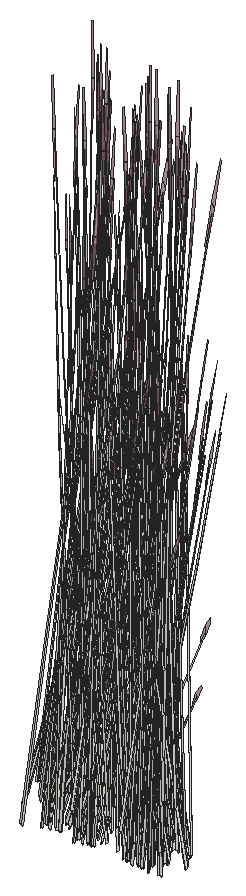
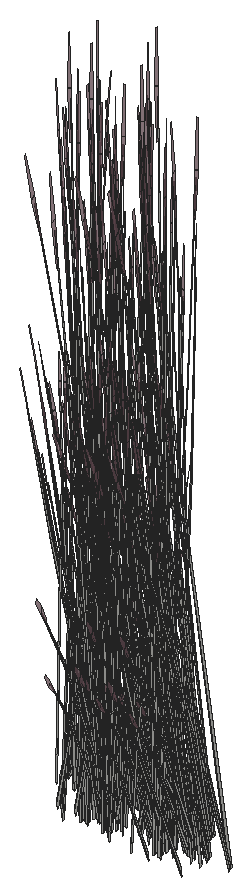
# SketchUp Ruby script. Lengths in inches.
U = 1.inch
M = Sketchup.active_model
def pt(a) = Geom::Point3d.new(a.map { |v| v * U })
def face(e, loops, mat)
  f = e.add_face(loops[0].map { |a| pt(a) })
  loops[1..].each { |l| e.add_face(l.map { |a| pt(a) }).erase! }
  f.material = f.back_material = mat if mat
  f
end
# faces: each face lists its corners as indices into pts; further lists are holes
def faces(e, pts, list, mat = nil) = list.each { |f| face(e, (f[0].is_a?(Array) ? f : [f]).map { |l| l.map { |i| pts[i] } }, mat) }
# xy, xz, yz: faces in a plane at the given z, y or x. An outline is a flat list of corners, or four numbers for a rectangle; further outlines are holes
def ring(l) = l.size == 4 ? [[l[0], l[1]], [l[2], l[1]], [l[2], l[3]], [l[0], l[3]]] : l.each_slice(2).to_a
def flat(e, list, mat, &to3) = list.each { |f| face(e, (f[0].is_a?(Array) ? f : [f]).map { |l| ring(l).map { |u, v| to3.(u, v) } }, mat) }
def xy(e, z, list, mat = nil) = flat(e, list, mat) { |x, y| [x, y, z] }
def xz(e, y, list, mat = nil) = flat(e, list, mat) { |x, z| [x, y, z] }
def yz(e, x, list, mat = nil) = flat(e, list, mat) { |y, z| [x, y, z] }
def lines(e, pts, list) = list.each { |a, b| e.add_line(pt(pts[a]), pt(pts[b])) }
# prism: a flat outline (further loops are holes) pulled along v
def prism(e, loops, v, mat = nil)
  f = face(e, loops, mat); d = Geom::Vector3d.new(v.map { |x| x * U })
  f.pushpull(f.normal.samedirection?(d) ? d.length : -d.length)
end
def box(e, o, s, mat = nil) = prism(e, [[o, [o[0] + s[0], o[1], o[2]], [o[0] + s[0], o[1] + s[1], o[2]], [o[0], o[1] + s[1], o[2]]]], [0, 0, s[2]], mat)
def at(x, y, z, deg = 0) = Geom::Transformation.translation(pt([x, y, z])) * Geom::Transformation.rotation(ORIGIN, Z_AXIS, deg.degrees)
def axes(o, x, y, z) = Geom::Transformation.new([*x, 0, *y, 0, *z, 0, *pt(o).to_a, 1])
def part(name) = M.definitions.add(name)
# library, detail: a bought-in or finely detailed component or shape, given as its bounding box
def library(name, o, s) = part(name).tap { |d| box(d.entities, o, s) }
def detail(e, o, s) = box(e.add_group.entities, o, s)
def put(e, d, t, mat = nil) = e.add_instance(d, t).tap { |i| i.material = mat if mat }
def group(e, t, mat = nil) = e.add_group.tap { |g| g.transformation = t; g.material = mat if mat }.entities
root = M.entities
M.materials.add("LightPink_Translucent").color = [144, 107, 117]
M.materials["LightPink_Translucent"].alpha = 0.75
c1 = part("blade")
p = [[2.15,0.21,22],[0,0.17,0],[0.09,0.45,0],[2.18,0.31,22],[2.29,0.31,22],[0.38,0.45,0],
  [2.48,0.24,33],[2.49,0.24,33],[2.48,0.22,33]]
faces(c1.entities,p,[[0,1,2,3],[4,5,2,3],[6,3,4,7],[8,0,3,6]])
c2 = part("seeds")
p = [[0.3,-0.1,1.38],[-0.01,-0.03,1.59],[-0.01,-0.03,0.03],[0.14,-0.07,-0.07],[0.29,-0.03,3],[0.15,0.01,3.11]]
faces(c2.entities,p,[[0,1,2,3],[1,0,4,5]],"LightPink_Translucent")
c3 = part("blade with seeds")
put(c3.entities,c1,at(0,0,0))
put(c3.entities,c2,axes([2.4,0.25,30.99],[1.5799,-0.05474,1.17369],[-0.12525,1.92788,0.29478],[-0.07173,-0.02425,1.56792]))
put(root,c3,axes([344.95,356.4,623.05],[-0.20082,-0.29199,0.35414],[0.2293,-0.2764,-0.4572],[0.1165,0.04206,0.87481]))
put(root,c3,axes([347.81,356.44,622.73],[-0.29004,-0.02173,0.0643],[0.00795,-0.32812,0.50621],[-0.03035,0.12569,0.77189]))
put(root,c3,axes([345.13,356.66,622.73],[-0.01777,0.35463,0.0643],[-0.26836,-0.00972,0.50621],[0.1028,0.03711,0.77189]))
put(root,c3,axes([343.93,356.03,620.59],[-0.085,-0.1147,1.43002],[0.1106,-0.37943,-0.30754],[0.17198,0.0514,0.61141]))
put(root,c3,axes([345.16,356.55,622.73],[-0.26024,0.30729,0.48003],[-0.22444,-0.32634,0.3958],[0.1221,0.05668,0.9933]))
put(root,c3,axes([347.375,355.65,620.03],[-0.24637,0.29097,-0.30978],[-0.24637,-0.29097,0.30978],[0,0.09372,1.38974]))
put(root,c3,axes([349.12,355.84,620.06],[-0.23773,0.35053,-0.62353],[-0.29532,-0.31785,-0.16365],[-0.09526,0.08744,1.37633]))
put(root,c3,axes([345.83,356.6,621.93],[-0.06755,-0.39203,-0.03492],[0.31928,-0.09013,-0.15832],[0.06667,0.02485,0.52218]))
put(root,c3,axes([346.67,355.6,620.09],[0.12941,0.42699,-0.69212],[-0.37279,0.15378,-0.18165],[0.0143,0.14459,1.52773]))
put(root,c3,axes([344.59,354.79,620.06],[0.36714,0.07646,-0.62353],[-0.07747,0.47163,-0.16365],[0.10956,0.05715,1.37633]))
put(root,c3,axes([346.625,355.09,620.62],[0.32884,-0.136,0.1448],[0.11516,0.38837,-0.41347],[0,0.08547,1.26744]))
put(root,c3,axes([346.51,355.12,620.67],[0.39748,0.22252,-0.29095],[-0.19139,0.46966,-0.50002],[0.01249,0.11531,1.59708]))
put(root,c3,axes([349.11,355.56,620.21],[-0.38326,0.02879,-0.44739],[-0.03466,-0.47788,0.21531],[-0.06861,0.04843,1.43643]))
put(root,c3,axes([344.51,355.8,621.875],[-0.1311,-0.08035,1.71376],[0.27131,-0.33708,0.13857],[0.16909,0.15206,0.73262]))
put(root,c3,axes([347.375,355.23,620.48],[0,-0.46636,0.49651],[0.39487,0,0],[0,0.10622,1.57504]))
put(root,c3,axes([347.54,355.66,620.02],[0,0.46636,-0.49651],[-0.39487,0,0],[0,0.10622,1.57504]))
put(root,c3,axes([345.23,356.55,622.53],[0.20082,0.29199,-0.35414],[-0.2293,0.2764,0.4572],[0.1165,0.04206,0.87481]))
put(root,c3,axes([345.01,356.59,623.03],[0.0189,-0.47427,-0.1216],[0.35781,0.01296,-0.67495],[0.13781,0.03295,1.02557]))
put(root,c3,axes([349.51,356.79,620.02],[-0.33032,0.23318,-0.49651],[-0.19744,-0.41812,0],[-0.07523,0.05311,1.57504]))
put(root,c3,axes([349.53,356.67,620.19],[-0.21791,-0.46895,-0.05142],[0.36918,-0.26061,0.51607],[-0.09097,0.04465,1.6363]))
put(root,c3,axes([349.44,356.61,620.03],[-0.32928,-0.11539,-0.30978],[0.08291,-0.40636,0.30978],[-0.06638,0.04686,1.38974]))
put(root,c3,axes([348.02,356.22,623.05],[0.23881,-0.24554,0.35414],[0.22606,0.28036,-0.4572],[-0.0344,0.14245,0.87481]))
put(root,c3,axes([349.625,354.87,620.84],[-0.00964,-0.43909,1.41272],[0.43635,0.11382,0.59816],[-0.1032,0.24027,1.3335]))
put(root,c3,axes([346.375,356.82,623.05],[-0.05451,-0.37564,0.35414],[0.31161,-0.09919,-0.4572],[0.0837,0.10765,0.87481]))
put(root,c3,axes([345.32,356.3,622.72],[0.07571,-0.00789,1.74944],[0.20767,-0.36231,-0.27667],[0.13467,0.04783,0.14031]))
put(root,c3,axes([346.44,354.85,620.21],[0.21202,0.39143,-0.44739],[-0.32115,0.27564,0.21531],[0.06861,0.04843,1.43643]))
put(root,c3,axes([349.38,355.43,620.67],[0.04113,0.53214,-0.29095],[-0.42835,0.03218,-0.50002],[-0.07543,0.07088,1.59708]))
put(root,c3,axes([346.58,354.66,622.47],[-0.30498,-0.24231,1.38283],[0.32203,-0.37727,0.59665],[0.0984,0.22736,1.33663]))
put(root,c3,axes([346.21,355.62,620.77],[-0.21807,0.07699,1.1486],[0.10265,-0.31819,0.84392],[0.11568,0.02177,0.25299]))
put(root,c3,axes([346.07,357.34,622.71],[0.00104,-0.05646,1.77383],[0.30246,-0.2491,-0.16761],[0.10506,0.08891,0.31391]))
put(root,c3,axes([347.04,356.63,620.77],[-0.19872,-0.13409,1.1486],[0.2566,-0.13625,0.84392],[0.06921,0.11541,0.25299]))
put(root,c3,axes([345.02,356.36,622.98],[0.35281,0.01123,-0.71045],[-0.0237,0.47284,0.08574],[0.14947,0.0499,1.00501]))
put(root,c3,axes([347.64,355.31,620.375],[0.44133,0,0],[0,0.52122,-0.51607],[0,0.11871,1.63711]))
put(root,c3,axes([346.11,356.96,622.71],[-0.03191,-0.04083,1.77383],[0.06981,-0.43764,-0.16761],[0.12571,-0.02796,0.31391]))
put(root,c3,axes([349.8125,356.72,620.375],[0.22066,0.46731,0],[-0.36918,0.26061,-0.51607],[-0.08408,0.05936,1.63711]))
put(root,c3,axes([346.35,357.01,623.03],[0.21031,-0.39918,-0.1216],[0.30457,0.22997,-0.67495],[0.10587,0.11278,1.02557]))
put(root,c3,axes([349.46,355.53,620.62],[0.26075,0.2802,0.1448],[-0.2175,0.31612,-0.41347],[-0.06054,0.04274,1.26744]))
put(root,c3,axes([352.03,354.77,621.875],[0.12246,-0.09864,1.71376],[0.1031,0.45582,0.13857],[-0.19225,0.10302,0.73262]))
put(root,c3,axes([349.45,355.33,620.72],[0.38326,-0.02879,0.44739],[0.03466,0.47788,-0.21531],[-0.06861,0.04843,1.43643]))
put(root,c3,axes([345.8,356.125,620.59],[-0.085,-0.1147,1.43002],[0.1106,-0.37943,-0.30754],[0.17198,0.0514,0.61141]))
put(root,c3,axes([351.65,355.55,620.59],[0.12266,0.03828,1.43002],[0.07906,0.39104,-0.30754],[-0.16661,0.0732,0.61141]))
put(root,c3,axes([349.54,356.43,620.33],[0.44186,0.15158,0.30756],[-0.11054,0.54181,-0.36492],[-0.07313,0.06781,1.64885]))
put(root,c3,axes([346.99,356.31,623.05],[-0.20082,-0.29199,0.35414],[0.2293,-0.2764,-0.4572],[0.1165,0.04206,0.87481]))
put(root,c3,axes([349.73,356.4,620.48],[0.33032,-0.23318,0.49651],[0.19744,0.41812,0],[-0.07523,0.05311,1.57504]))
put(root,c3,axes([347.18,356.57,622.73],[-0.01777,0.35463,0.0643],[-0.26836,-0.00972,0.50621],[0.1028,0.03711,0.77189]))
put(root,c3,axes([347.1,357.13,619.49],[0.02571,-0.06733,1.76342],[0.32373,-0.19829,-0.26939],[0.09815,0.10263,0.30037]))
put(root,c3,axes([347.2,356.46,622.73],[-0.26024,0.30729,0.48003],[-0.22444,-0.32634,0.3958],[0.1221,0.05668,0.9933]))
put(root,c3,axes([347.88,356.51,621.93],[-0.06755,-0.39203,-0.03492],[0.31928,-0.09013,-0.15832],[0.06667,0.02485,0.52218]))
put(root,c3,axes([349.54,355.22,620.21],[-0.17124,0.42022,-0.44739],[-0.35581,-0.20224,0.21531],[0,0.09687,1.43643]))
put(root,c3,axes([349.48,354.98,620.29],[0,0.53934,-0.05637],[-0.44133,0,0],[0,0.01695,1.79368]))
put(root,c3,axes([348.69,356.625,623.05],[0.1064,-0.35863,0.35414],[0.31043,0.1046,-0.4572],[0.02846,0.14439,0.87481]))
put(root,c3,axes([351.02,355.06,622.71],[0.04504,0.01251,1.77383],[0.13934,0.41205,-0.16761],[-0.0922,0.10815,0.31391]))
put(root,c3,axes([346.56,355.71,621.875],[-0.1311,-0.08035,1.71376],[0.27131,-0.33708,0.13857],[0.16909,0.15206,0.73262]))
put(root,c3,axes([349.26,356.03,620.29],[0.15345,0.53576,-0.06012],[-0.43845,0.18773,0],[0.00536,0.01871,1.72173]))
put(root,c3,axes([347.28,356.46,622.53],[0.20082,0.29199,-0.35414],[-0.2293,0.2764,0.4572],[0.1165,0.04206,0.87481]))
put(root,c3,axes([350.53,355.33,620.2],[-0.44111,-0.00373,-0.04976],[0,-0.52122,0.49943],[-0.01386,0.11865,1.58352]))
put(root,c3,axes([347.05,356.5,623.03],[0.0189,-0.47427,-0.1216],[0.35781,0.01296,-0.67495],[0.13781,0.03295,1.02557]))
put(root,c3,axes([351.4,356.37,620.77],[0.14709,-0.21136,1.1486],[0.05804,0.3346,0.84392],[-0.1063,0.05991,0.25299]))
put(root,c3,axes([349.39,356.2,620.2],[0.35581,0.20937,0],[-0.17124,0.43505,0],[0,0,1.74954]))
put(root,c3,axes([352.48,355.08,621.875],[0.08815,-0.14329,1.71376],[0.22258,0.38678,0.13857],[-0.15267,0.17614,0.73262]))
put(root,c3,axes([351.95,355.45,622.53],[-0.30722,0.06665,-0.35414],[-0.08112,-0.381,0.4572],[-0.08804,0.10234,0.87481]))
put(root,c3,axes([347.36,356.21,622.72],[0.07571,-0.00789,1.74944],[0.20767,-0.36231,-0.27667],[0.13467,0.04783,0.14031]))
put(root,c3,axes([351.78,356.59,619.49],[0.04734,0.04659,1.76342],[0.08027,0.4317,-0.26939],[-0.10492,0.09206,0.30037]))
put(root,c3,axes([350.44,355.4,620.03],[-0.24637,0.29097,-0.30978],[-0.24637,-0.29097,0.30978],[0,0.09372,1.38974]))
put(root,c3,axes([348.26,355.53,620.77],[-0.21807,0.07699,1.1486],[0.10265,-0.31819,0.84392],[0.11568,0.02177,0.25299]))
put(root,c3,axes([351.99,355.37,622.73],[-0.08753,-0.42921,0.48003],[0.34336,-0.07449,0.3958],[-0.1012,0.10094,0.9933]))
put(root,c3,axes([349.74,355.35,620.09],[0.12941,0.42699,-0.69212],[-0.37279,0.15378,-0.18165],[0.0143,0.14459,1.52773]))
put(root,c3,axes([349.69,354.84,620.62],[0.32884,-0.136,0.1448],[0.11516,0.38837,-0.41347],[0,0.08547,1.26744]))
put(root,c3,axes([351.92,355.29,622.73],[-0.2423,-0.19613,0.0643],[0.14107,-0.2793,0.50621],[-0.07768,0.0903,0.77189]))
put(root,c3,axes([347.07,356.27,622.98],[0.35281,0.01123,-0.71045],[-0.0237,0.47284,0.08574],[0.14947,0.0499,1.00501]))
put(root,c3,axes([349.58,354.87,620.67],[0.39748,0.22252,-0.29095],[-0.19139,0.46966,-0.50002],[0.01249,0.11531,1.59708]))
put(root,c3,axes([348.15,356.87,622.71],[-0.03191,-0.04083,1.77383],[0.06981,-0.43764,-0.16761],[0.12571,-0.02796,0.31391]))
put(root,c3,axes([352.21,355.5,622.68],[0.09067,0.42583,-0.51099],[-0.34336,0.07449,-0.3958],[-0.0984,0.11438,0.97773]))
put(root,c3,axes([350.44,354.98,620.48],[0,-0.46636,0.49651],[0.39487,0,0],[0,0.10622,1.57504]))
put(root,c3,axes([350.61,355.41,620.02],[0,0.46636,-0.49651],[-0.39487,0,0],[0,0.10622,1.57504]))
put(root,c3,axes([352.04,355.19,623.03],[0.32648,0.25715,-0.1216],[-0.18809,0.3724,-0.67495],[-0.09224,0.12945,1.02557]))
put(root,c3,axes([347.85,356.04,620.59],[-0.085,-0.1147,1.43002],[0.1106,-0.37943,-0.30754],[0.17198,0.0514,0.61141]))
put(root,c3,axes([354.19,354.5,621.875],[0.12246,-0.09864,1.71376],[0.1031,0.45582,0.13857],[-0.19225,0.10302,0.73262]))
put(root,c3,axes([349.4375,356.57,623.05],[-0.05451,-0.37564,0.35414],[0.31161,-0.09919,-0.4572],[0.0837,0.10765,0.87481]))
put(root,c3,axes([353.81,355.28,620.59],[0.12266,0.03828,1.43002],[0.07906,0.39104,-0.30754],[-0.16661,0.0732,0.61141]))
put(root,c3,axes([349.51,354.6,620.21],[0.21202,0.39143,-0.44739],[-0.32115,0.27564,0.21531],[0.06861,0.04843,1.43643]))
put(root,c3,axes([351.5,356.3125,623.65],[0.31145,0.12449,-0.06488],[-0.0958,0.38314,-0.29416],[-0.05094,0.05817,0.97024]))
put(root,c3,axes([349.65,354.41,622.47],[-0.30498,-0.24231,1.38283],[0.32203,-0.37727,0.59665],[0.0984,0.22736,1.33663]))
put(root,c3,axes([352.2,355.23,623.05],[0.30722,-0.06665,0.35414],[0.08112,0.381,-0.4572],[-0.08804,0.10234,0.87481]))
put(root,c3,axes([349.13,357.09,622.71],[0.00104,-0.05646,1.77383],[0.30246,-0.2491,-0.16761],[0.10506,0.08891,0.31391]))
put(root,c3,axes([350.11,356.38,620.77],[-0.19872,-0.13409,1.1486],[0.2566,-0.13625,0.84392],[0.06921,0.11541,0.25299]))
put(root,c3,axes([350.71,355.06,620.375],[0.44133,0,0],[0,0.52122,-0.51607],[0,0.11871,1.63711]))
put(root,c3,axes([352.49,356.24,622.73],[-0.25132,-0.3182,0.48003],[0.2669,-0.27442,0.3958],[-0.04636,0.14929,0.9933]))
put(root,c3,axes([352.4,356.21,622.73],[-0.29004,-0.02173,0.0643],[0.00795,-0.32812,0.50621],[-0.03035,0.12569,0.77189]))
put(root,c3,axes([350.14,356.99,620.67],[-0.22633,-0.01463,1.0506],[0.14947,-0.31064,0.58006],[0.08941,0.11036,0.8241]))
put(root,c3,axes([353.71,355.6,620.06],[-0.23773,0.35053,-0.62353],[-0.29532,-0.31785,-0.16365],[-0.09526,0.08744,1.37633]))
put(root,c3,axes([353.18,354.79,622.71],[0.04504,0.01251,1.77383],[0.13934,0.41205,-0.16761],[-0.0922,0.10815,0.31391]))
put(root,c3,axes([349.41,356.76,623.03],[0.21031,-0.39918,-0.1216],[0.30457,0.22997,-0.67495],[0.10587,0.11278,1.02557]))
put(root,c3,axes([353.55,356.09,620.77],[0.14709,-0.21136,1.1486],[0.05804,0.3346,0.84392],[-0.1063,0.05991,0.25299]))
put(root,c3,axes([349.66,356.5625,622.68],[0.34827,-0.11086,-0.51099],[0.06092,0.41983,-0.3958],[0.09354,0.12031,0.97773]))
put(root,c3,axes([353.7,355.32,620.21],[-0.38326,0.02879,-0.44739],[-0.03466,-0.47788,0.21531],[-0.06861,0.04843,1.43643]))
put(root,c3,axes([350.06,356.06,623.05],[-0.20082,-0.29199,0.35414],[0.2293,-0.2764,-0.4572],[0.1165,0.04206,0.87481]))
put(root,c3,axes([350.24,356.32,622.73],[-0.01777,0.35463,0.0643],[-0.26836,-0.00972,0.50621],[0.1028,0.03711,0.77189]))
put(root,c3,axes([350.16,356.875,619.49],[0.02571,-0.06733,1.76342],[0.32373,-0.19829,-0.26939],[0.09815,0.10263,0.30037]))
put(root,c3,axes([354.64,354.81,621.875],[0.08815,-0.14329,1.71376],[0.22258,0.38678,0.13857],[-0.15267,0.17614,0.73262]))
put(root,c3,axes([354.11,355.18,622.53],[-0.30722,0.06665,-0.35414],[-0.08112,-0.381,0.4572],[-0.08804,0.10234,0.87481]))
put(root,c3,axes([350.27,356.21,622.73],[-0.26024,0.30729,0.48003],[-0.22444,-0.32634,0.3958],[0.1221,0.05668,0.9933]))
put(root,c3,axes([350.94,356.26,621.93],[-0.06755,-0.39203,-0.03492],[0.31928,-0.09013,-0.15832],[0.06667,0.02485,0.52218]))
put(root,c3,axes([353.94,356.3125,619.49],[0.04734,0.04659,1.76342],[0.08027,0.4317,-0.26939],[-0.10492,0.09206,0.30037]))
put(root,c3,axes([354.11,356.56,620.02],[-0.33032,0.23318,-0.49651],[-0.19744,-0.41812,0],[-0.07523,0.05311,1.57504]))
put(root,c3,axes([354.13,356.43,620.19],[-0.21791,-0.46895,-0.05142],[0.36918,-0.26061,0.51607],[-0.09097,0.04465,1.6363]))
put(root,c3,axes([354.15,355.1,622.73],[-0.08753,-0.42921,0.48003],[0.34336,-0.07449,0.3958],[-0.1012,0.10094,0.9933]))
put(root,c3,axes([354.08,355.02,622.73],[-0.2423,-0.19613,0.0643],[0.14107,-0.2793,0.50621],[-0.07768,0.0903,0.77189]))
put(root,c3,axes([354.03,356.37,620.03],[-0.32928,-0.11539,-0.30978],[0.08291,-0.40636,0.30978],[-0.06638,0.04686,1.38974]))
put(root,c3,axes([352.62,355.99,623.05],[0.23881,-0.24554,0.35414],[0.22606,0.28036,-0.4572],[-0.0344,0.14245,0.87481]))
put(root,c3,axes([354.22,354.64,620.84],[-0.00964,-0.43909,1.41272],[0.43635,0.11382,0.59816],[-0.1032,0.24027,1.3335]))
put(root,c3,axes([354.57,355.16,621.875],[0.06572,-0.16029,1.71376],[0.27569,0.33172,0.13857],[-0.12437,0.20675,0.73262]))
put(root,c3,axes([349.62,355.46,621.875],[-0.1311,-0.08035,1.71376],[0.27131,-0.33708,0.13857],[0.16909,0.15206,0.73262]))
put(root,c3,axes([353.97,355.19,620.67],[0.04113,0.53214,-0.29095],[-0.42835,0.03218,-0.50002],[-0.07543,0.07088,1.59708]))
put(root,c3,axes([354.36,355.22,622.68],[0.09067,0.42583,-0.51099],[-0.34336,0.07449,-0.3958],[-0.0984,0.11438,0.97773]))
put(root,c3,axes([350.34,356.21,622.53],[0.20082,0.29199,-0.35414],[-0.2293,0.2764,0.4572],[0.1165,0.04206,0.87481]))
put(root,c3,axes([350.11,356.25,623.03],[0.0189,-0.47427,-0.1216],[0.35781,0.01296,-0.67495],[0.13781,0.03295,1.02557]))
put(root,c3,axes([354.2,354.92,623.03],[0.32648,0.25715,-0.1216],[-0.18809,0.3724,-0.67495],[-0.09224,0.12945,1.02557]))
put(root,c3,axes([350.43,355.96,622.72],[0.07571,-0.00789,1.74944],[0.20767,-0.36231,-0.27667],[0.13467,0.04783,0.14031]))
put(root,c3,axes([354.41,356.49,620.375],[0.22066,0.46731,0],[-0.36918,0.26061,-0.51607],[-0.08408,0.05936,1.63711]))
put(root,c3,axes([353.66,356.04,623.65],[0.31145,0.12449,-0.06488],[-0.0958,0.38314,-0.29416],[-0.05094,0.05817,0.97024]))
put(root,c3,axes([354.36,354.95,623.05],[0.30722,-0.06665,0.35414],[0.08112,0.381,-0.4572],[-0.08804,0.10234,0.87481]))
put(root,c3,axes([354.05,355.3,620.62],[0.26075,0.2802,0.1448],[-0.2175,0.31612,-0.41347],[-0.06054,0.04274,1.26744]))
put(root,c3,axes([350.13,356.02,622.98],[0.35281,0.01123,-0.71045],[-0.0237,0.47284,0.08574],[0.14947,0.0499,1.00501]))
put(root,c3,axes([354.04,355.09,620.72],[0.38326,-0.02879,0.44739],[0.03466,0.47788,-0.21531],[-0.06861,0.04843,1.43643]))
put(root,c3,axes([354.14,356.19,620.33],[0.44186,0.15158,0.30756],[-0.11054,0.54181,-0.36492],[-0.07313,0.06781,1.64885]))
put(root,c3,axes([351.22,356.62,622.71],[-0.03191,-0.04083,1.77383],[0.06981,-0.43764,-0.16761],[0.12571,-0.02796,0.31391]))
put(root,c3,axes([354.33,356.16,620.48],[0.33032,-0.23318,0.49651],[0.19744,0.41812,0],[-0.07523,0.05311,1.57504]))
put(root,c3,axes([354.65,355.97,622.73],[-0.25132,-0.3182,0.48003],[0.2669,-0.27442,0.3958],[-0.04636,0.14929,0.9933]))
put(root,c3,axes([354.56,355.9375,622.73],[-0.29004,-0.02173,0.0643],[0.00795,-0.32812,0.50621],[-0.03035,0.12569,0.77189]))
put(root,c3,axes([357.01,355.4,621.875],[0.12246,-0.09864,1.71376],[0.1031,0.45582,0.13857],[-0.19225,0.10302,0.73262]))
put(root,c3,axes([355.87,355.33,620.06],[-0.23773,0.35053,-0.62353],[-0.29532,-0.31785,-0.16365],[-0.09526,0.08744,1.37633]))
put(root,c3,axes([356.63,356.18,620.59],[0.12266,0.03828,1.43002],[0.07906,0.39104,-0.30754],[-0.16661,0.0732,0.61141]))
put(root,c3,axes([354.13,354.99,620.21],[-0.17124,0.42022,-0.44739],[-0.35581,-0.20224,0.21531],[0,0.09687,1.43643]))
put(root,c3,axes([350.91,355.79,620.59],[-0.085,-0.1147,1.43002],[0.1106,-0.37943,-0.30754],[0.17198,0.0514,0.61141]))
put(root,c3,axes([357.71,354.93,621.34],[0.10032,-0.06746,1.77064],[0.0346,0.47103,0.13857],[-0.2173,0.0625,0.63284]))
put(root,c3,axes([353.29,356.39,623.05],[0.1064,-0.35863,0.35414],[0.31043,0.1046,-0.4572],[0.02846,0.14439,0.87481]))
put(root,c3,axes([353.86,355.79,620.29],[0.15345,0.53576,-0.06012],[-0.43845,0.18773,0],[0.00536,0.01871,1.72173]))
put(root,c3,axes([356.64,355.24,622.72],[-0.05763,0.06055,1.74944],[0.0049,0.44239,-0.27667],[-0.13211,0.05753,0.14031]))
put(root,c3,axes([355.125,355.09,620.2],[-0.44111,-0.00373,-0.04976],[0,-0.52122,0.49943],[-0.01386,0.11865,1.58352]))
put(root,c3,axes([356.26,356.28,620.02],[-0.33032,0.23318,-0.49651],[-0.19744,-0.41812,0],[-0.07523,0.05311,1.57504]))
put(root,c3,axes([353.7,357.67,623.65],[0.2439,-0.26754,-0.06488],[0.22348,0.29302,-0.29416],[0.01573,0.08303,0.97024]))
put(root,c3,axes([356.28,356.16,620.19],[-0.21791,-0.46895,-0.05142],[0.36918,-0.26061,0.51607],[-0.09097,0.04465,1.6363]))
put(root,c3,axes([356,355.6875,622.71],[0.04504,0.01251,1.77383],[0.13934,0.41205,-0.16761],[-0.0922,0.10815,0.31391]))
put(root,c3,axes([357.02,355.18,622.68],[-0.09562,0.42421,-0.51099],[-0.32782,-0.1454,-0.3958],[-0.13199,0.0389,0.97773]))
put(root,c3,axes([353.99,355.97,620.2],[0.35581,0.20937,0],[-0.17124,0.43505,0],[0,0,1.74954]))
put(root,c3,axes([356.19,356.1,620.03],[-0.32928,-0.11539,-0.30978],[0.08291,-0.40636,0.30978],[-0.06638,0.04686,1.38974]))
put(root,c3,axes([354.77,355.71,623.05],[0.23881,-0.24554,0.35414],[0.22606,0.28036,-0.4572],[-0.0344,0.14245,0.87481]))
put(root,c3,axes([356.375,354.36,620.84],[-0.00964,-0.43909,1.41272],[0.43635,0.11382,0.59816],[-0.1032,0.24027,1.3335]))
put(root,c3,axes([355.03,355.17,620.03],[-0.24637,0.29097,-0.30978],[-0.24637,-0.29097,0.30978],[0,0.09372,1.38974]))
put(root,c3,axes([356.375,357,620.77],[0.14709,-0.21136,1.1486],[0.05804,0.3346,0.84392],[-0.1063,0.05991,0.25299]))
put(root,c3,axes([354.33,355.11,620.09],[0.12941,0.42699,-0.69212],[-0.37279,0.15378,-0.18165],[0.0143,0.14459,1.52773]))
put(root,c3,axes([356.13,354.92,620.67],[0.04113,0.53214,-0.29095],[-0.42835,0.03218,-0.50002],[-0.07543,0.07088,1.59708]))
put(root,c3,axes([354.28,354.61,620.62],[0.32884,-0.136,0.1448],[0.11516,0.38837,-0.41347],[0,0.08547,1.26744]))
put(root,c3,axes([357.01,354.82,623.03],[0.17758,0.42229,-0.1216],[-0.31518,0.20752,-0.67495],[-0.13282,0.05572,1.02557]))
put(root,c3,axes([357.46,355.71,621.875],[0.08815,-0.14329,1.71376],[0.22258,0.38678,0.13857],[-0.15267,0.17614,0.73262]))
put(root,c3,axes([356.93,356.08,622.53],[-0.30722,0.06665,-0.35414],[-0.08112,-0.381,0.4572],[-0.08804,0.10234,0.87481]))
put(root,c3,axes([354.17,354.64,620.67],[0.39748,0.22252,-0.29095],[-0.19139,0.46966,-0.50002],[0.01249,0.11531,1.59708]))
put(root,c3,axes([356.97,356,622.73],[-0.08753,-0.42921,0.48003],[0.34336,-0.07449,0.3958],[-0.1012,0.10094,0.9933]))
put(root,c3,axes([355.03,354.74,620.48],[0,-0.46636,0.49651],[0.39487,0,0],[0,0.10622,1.57504]))
put(root,c3,axes([355.2,355.18,620.02],[0,0.46636,-0.49651],[-0.39487,0,0],[0,0.10622,1.57504]))
put(root,c3,axes([354.15,356.59,622.73],[-0.35104,0.10702,0.48003],[-0.06092,-0.41983,0.3958],[0.08256,0.12373,0.9933]))
put(root,c3,axes([354.08,356.67,622.73],[-0.16041,0.29625,0.0643],[-0.22843,-0.17248,0.50621],[0.07385,0.09498,0.77189]))
put(root,c3,axes([356.9,355.92,622.73],[-0.2423,-0.19613,0.0643],[0.14107,-0.2793,0.50621],[-0.07768,0.0903,0.77189]))
put(root,c3,axes([358.55,355.41,621.875],[0.12246,-0.09864,1.71376],[0.1031,0.45582,0.13857],[-0.19225,0.10302,0.73262]))
put(root,c3,axes([356.5625,356.21,620.375],[0.22066,0.46731,0],[-0.36918,0.26061,-0.51607],[-0.08408,0.05936,1.63711]))
put(root,c3,axes([358.17,356.19,620.59],[0.12266,0.03828,1.43002],[0.07906,0.39104,-0.30754],[-0.16661,0.0732,0.61141]))
put(root,c3,axes([356.21,355.02,620.62],[0.26075,0.2802,0.1448],[-0.2175,0.31612,-0.41347],[-0.06054,0.04274,1.26744]))
put(root,c3,axes([357.18,356.13,622.68],[0.09067,0.42583,-0.51099],[-0.34336,0.07449,-0.3958],[-0.0984,0.11438,0.97773]))
put(root,c3,axes([359.25,354.9375,621.34],[0.10032,-0.06746,1.77064],[0.0346,0.47103,0.13857],[-0.2173,0.0625,0.63284]))
put(root,c3,axes([354.03,356.33,623.05],[-0.05451,-0.37564,0.35414],[0.31161,-0.09919,-0.4572],[0.0837,0.10765,0.87481]))
put(root,c3,axes([356.29,355.92,620.33],[0.44186,0.15158,0.30756],[-0.11054,0.54181,-0.36492],[-0.07313,0.06781,1.64885]))
put(root,c3,axes([356.48,355.89,620.48],[0.33032,-0.23318,0.49651],[0.19744,0.41812,0],[-0.07523,0.05311,1.57504]))
put(root,c3,axes([354.24,354.17,622.47],[-0.30498,-0.24231,1.38283],[0.32203,-0.37727,0.59665],[0.0984,0.22736,1.33663]))
put(root,c3,axes([353.73,356.86,622.71],[0.00104,-0.05646,1.77383],[0.30246,-0.2491,-0.16761],[0.10506,0.08891,0.31391]))
put(root,c3,axes([358.17,355.25,622.72],[-0.05763,0.06055,1.74944],[0.0049,0.44239,-0.27667],[-0.13211,0.05753,0.14031]))
put(root,c3,axes([354.7,356.14,620.77],[-0.19872,-0.13409,1.1486],[0.2566,-0.13625,0.84392],[0.06921,0.11541,0.25299]))
put(root,c3,axes([357.02,355.82,623.03],[0.32648,0.25715,-0.1216],[-0.18809,0.3724,-0.67495],[-0.09224,0.12945,1.02557]))
put(root,c3,axes([357.76,357,620.375],[-0.22066,0.46731,0],[-0.36918,-0.26061,-0.51607],[-0.08408,-0.05936,1.63711]))
put(root,c3,axes([355.3,354.82,620.375],[0.44133,0,0],[0,0.52122,-0.51607],[0,0.11871,1.63711]))
put(root,c3,axes([357.53,355.7,622.71],[0.04504,0.01251,1.77383],[0.13934,0.41205,-0.16761],[-0.0922,0.10815,0.31391]))
put(root,c3,axes([358.56,355.19,622.68],[-0.09562,0.42421,-0.51099],[-0.32782,-0.1454,-0.3958],[-0.13199,0.0389,0.97773]))
put(root,c3,axes([356.28,354.71,620.21],[-0.17124,0.42022,-0.44739],[-0.35581,-0.20224,0.21531],[0,0.09687,1.43643]))
put(root,c3,axes([356.48,356.9375,623.65],[0.31145,0.12449,-0.06488],[-0.0958,0.38314,-0.29416],[-0.05094,0.05817,0.97024]))
put(root,c3,axes([357.18,355.86,623.05],[0.30722,-0.06665,0.35414],[0.08112,0.381,-0.4572],[-0.08804,0.10234,0.87481]))
put(root,c3,axes([354.73,356.75,620.67],[-0.22633,-0.01463,1.0506],[0.14947,-0.31064,0.58006],[0.08941,0.11036,0.8241]))
put(root,c3,axes([355.44,356.12,623.05],[0.1064,-0.35863,0.35414],[0.31043,0.1046,-0.4572],[0.02846,0.14439,0.87481]))
put(root,c3,axes([357.91,357.01,620.77],[0.14709,-0.21136,1.1486],[0.05804,0.3346,0.84392],[-0.1063,0.05991,0.25299]))
put(root,c3,axes([356.01,355.52,620.29],[0.15345,0.53576,-0.06012],[-0.43845,0.18773,0],[0.00536,0.01871,1.72173]))
put(root,c3,axes([354,356.53,623.03],[0.21031,-0.39918,-0.1216],[0.30457,0.22997,-0.67495],[0.10587,0.11278,1.02557]))
put(root,c3,axes([358.54,354.83,623.03],[0.17758,0.42229,-0.1216],[-0.31518,0.20752,-0.67495],[-0.13282,0.05572,1.02557]))
put(root,c3,axes([357.28,354.82,620.2],[-0.44111,-0.00373,-0.04976],[0,-0.52122,0.49943],[-0.01386,0.11865,1.58352]))
put(root,c3,axes([358.99,355.72,621.875],[0.08815,-0.14329,1.71376],[0.22258,0.38678,0.13857],[-0.15267,0.17614,0.73262]))
put(root,c3,axes([358.46,356.1,622.53],[-0.30722,0.06665,-0.35414],[-0.08112,-0.381,0.4572],[-0.08804,0.10234,0.87481]))
put(root,c3,axes([354.25,356.33,622.68],[0.34827,-0.11086,-0.51099],[0.06092,0.41983,-0.3958],[0.09354,0.12031,0.97773]))
